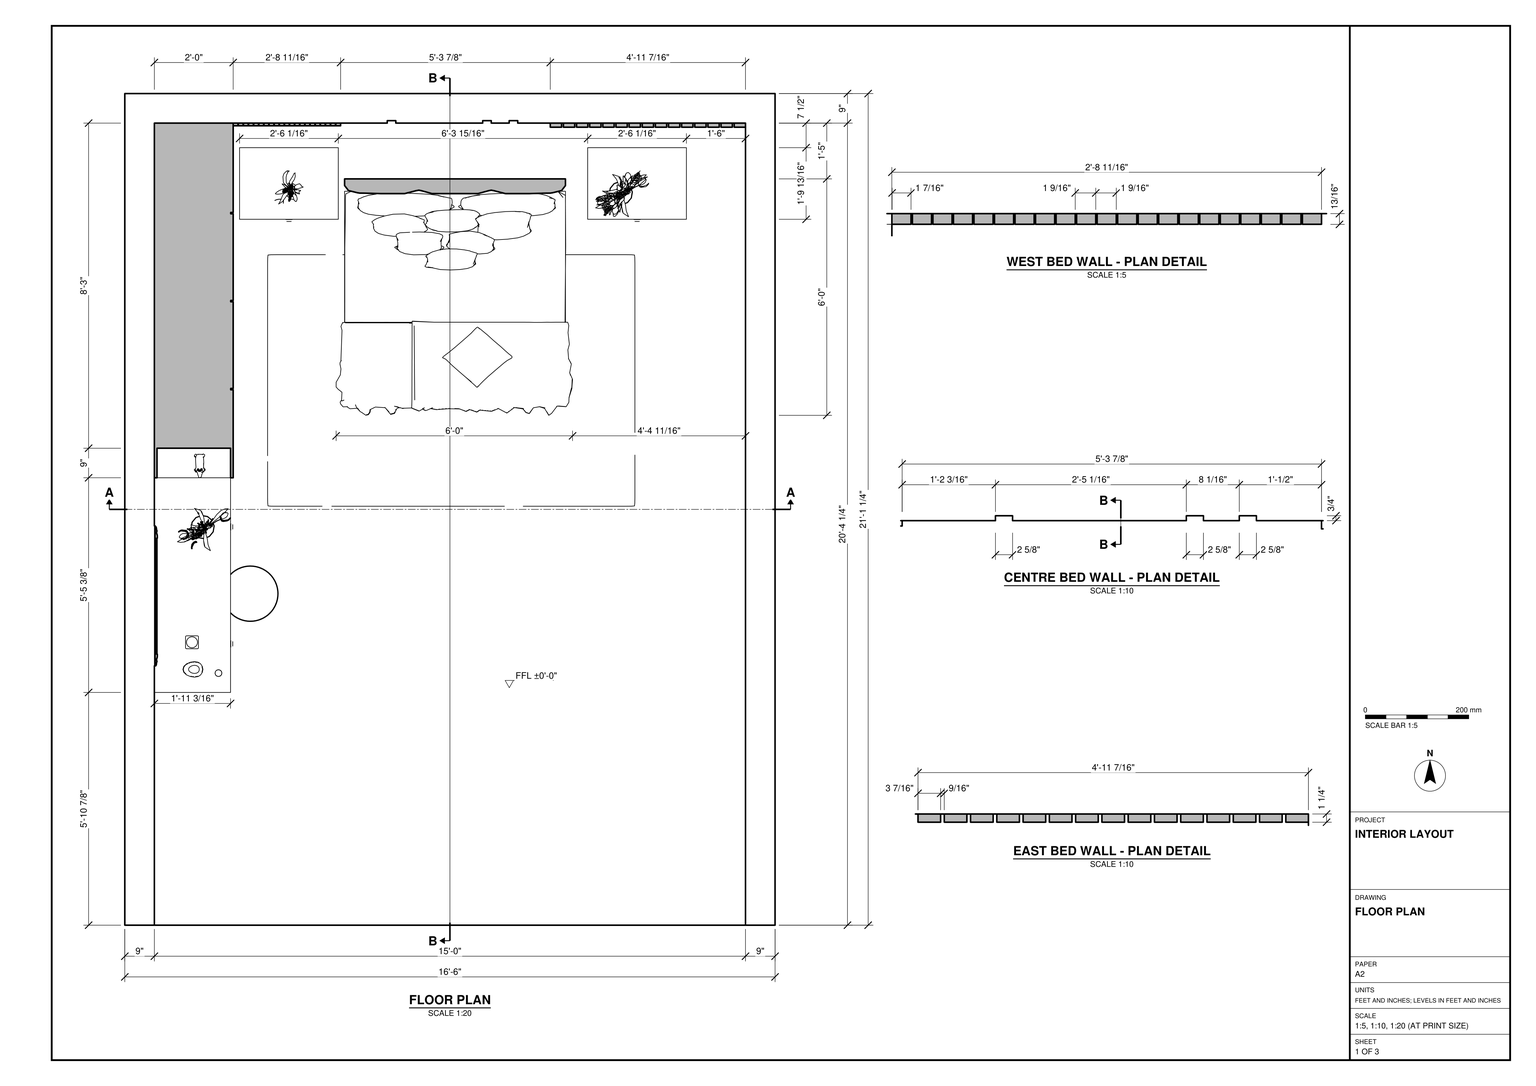
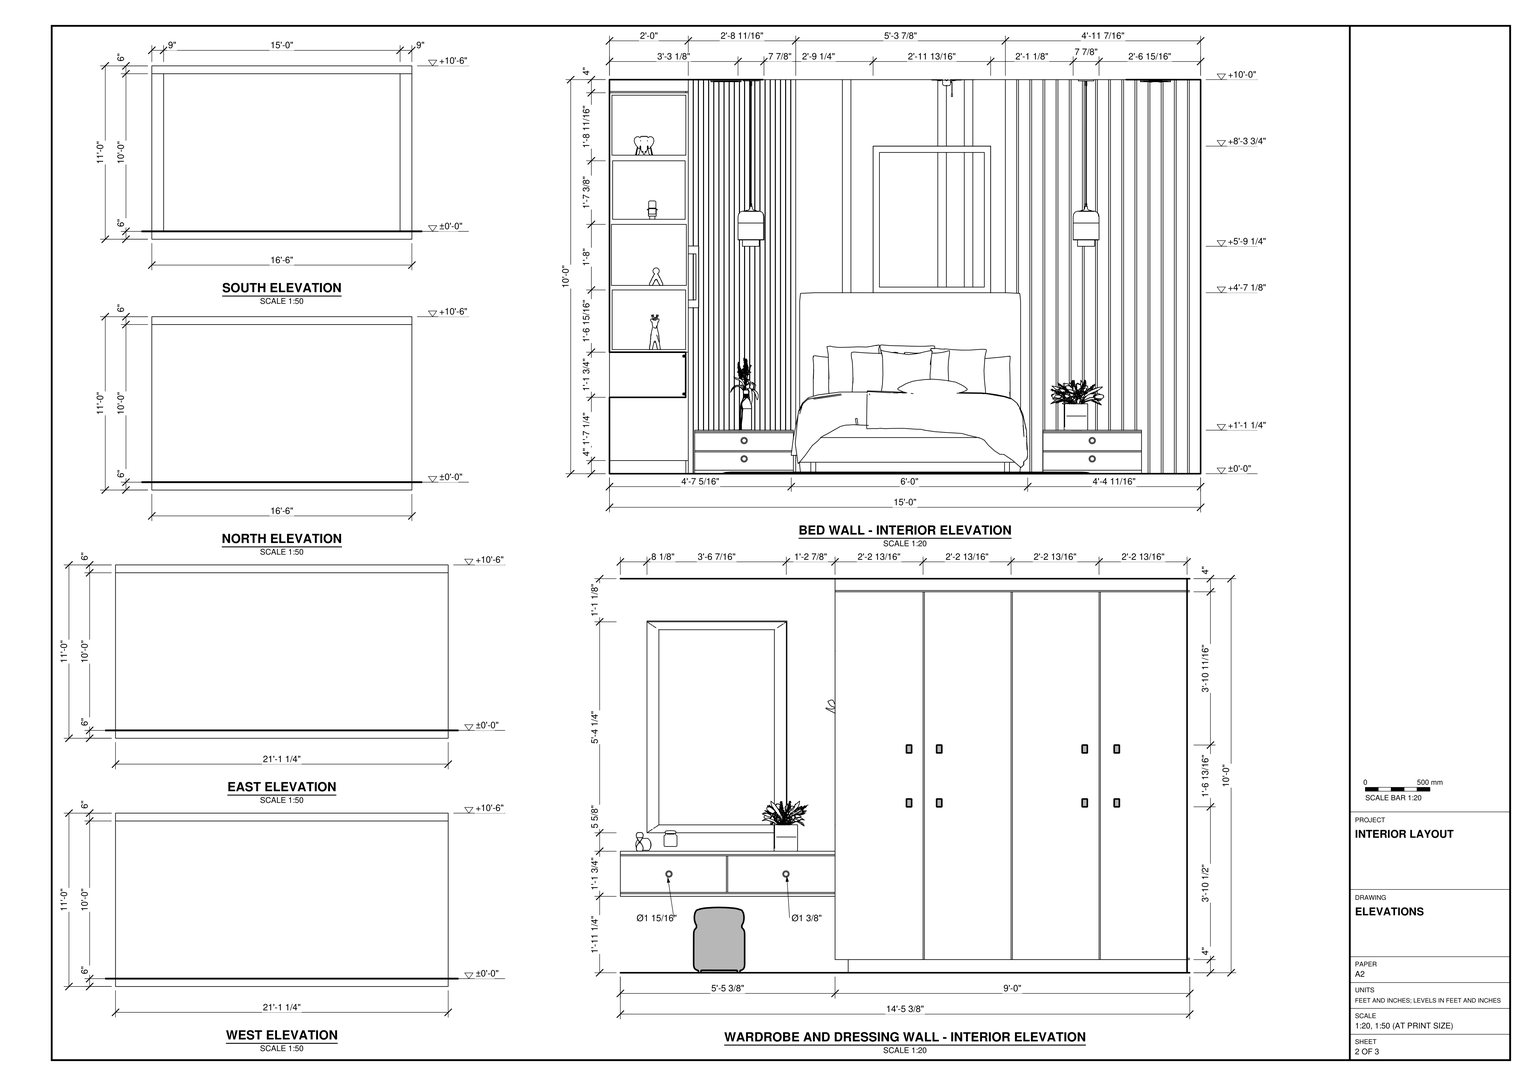
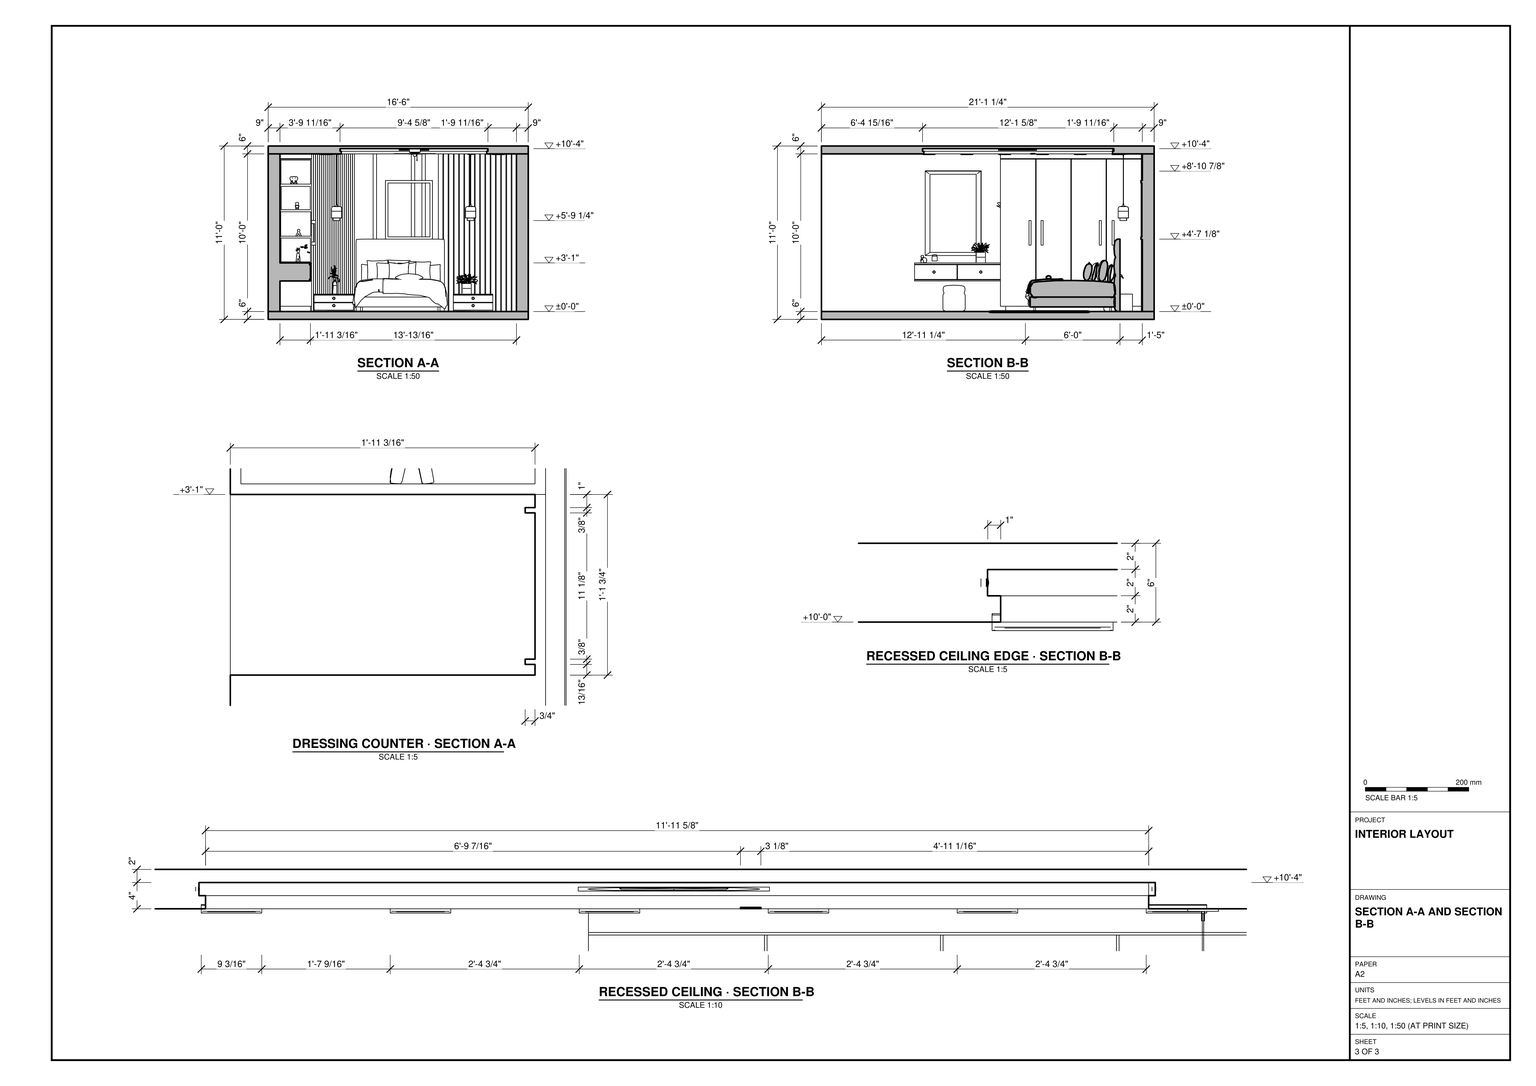
Model the bedroom in SketchUp from task_files/diagram_01.pdf. Work in feet and inches. The room shell measures 16'-6" across, 21'-1 1/4" from south to north and 11'-0" in overall height. Set the single finished floor at ±0'-0". Model the 9" walls on the north, east and west sides, leaving the south side open as shown in section. Include the 6" floor and roof slabs and form the stepped edge of the ceiling recess to match the section detail.

Place the bed with its headboard toward the north wall and a low drawer unit on either side. Use the bed-wall plan details to distinguish the closely spaced vertical strips on the west from the wider strips on the east. Model the central panel and its framed rectangular feature above the headboard. Along the west wall, build the tall wardrobe with its door fronts, handles and end display shelves. Continue the run toward the south with a wall-mounted dressing counter, drawers, a mirror above and a stool below. Keep the floor beyond the dressing area clear as shown in plan. Decor and loose items, including the rug, plants, pendant lights and shelf objects, may be any suitable library components.

Organise the walls, slabs and roof, and each furniture or joinery piece, as separate groups or components. Use components for repeated parts. Save one SketchUp model as output_files/bedroom_with_a_panelled_bed_wall_and_dressing_area.skp.

# SketchUp Ruby script. Lengths in inches.
U = 1.inch
M = Sketchup.active_model
def pt(a) = Geom::Point3d.new(a.map { |v| v * U })
def face(e, loops, mat)
  f = e.add_face(loops[0].map { |a| pt(a) })
  loops[1..].each { |l| e.add_face(l.map { |a| pt(a) }).erase! }
  f.material = f.back_material = mat if mat
  f
end
# faces: each face lists its corners as indices into pts; further lists are holes
def faces(e, pts, list, mat = nil) = list.each { |f| face(e, (f[0].is_a?(Array) ? f : [f]).map { |l| l.map { |i| pts[i] } }, mat) }
# xy, xz, yz: faces in a plane at the given z, y or x. An outline is a flat list of corners, or four numbers for a rectangle; further outlines are holes
def ring(l) = l.size == 4 ? [[l[0], l[1]], [l[2], l[1]], [l[2], l[3]], [l[0], l[3]]] : l.each_slice(2).to_a
def flat(e, list, mat, &to3) = list.each { |f| face(e, (f[0].is_a?(Array) ? f : [f]).map { |l| ring(l).map { |u, v| to3.(u, v) } }, mat) }
def xy(e, z, list, mat = nil) = flat(e, list, mat) { |x, y| [x, y, z] }
def xz(e, y, list, mat = nil) = flat(e, list, mat) { |x, z| [x, y, z] }
def yz(e, x, list, mat = nil) = flat(e, list, mat) { |y, z| [x, y, z] }
def lines(e, pts, list) = list.each { |a, b| e.add_line(pt(pts[a]), pt(pts[b])) }
# prism: a flat outline (further loops are holes) pulled along v
def prism(e, loops, v, mat = nil)
  f = face(e, loops, mat); d = Geom::Vector3d.new(v.map { |x| x * U })
  f.pushpull(f.normal.samedirection?(d) ? d.length : -d.length)
end
def box(e, o, s, mat = nil) = prism(e, [[o, [o[0] + s[0], o[1], o[2]], [o[0] + s[0], o[1] + s[1], o[2]], [o[0], o[1] + s[1], o[2]]]], [0, 0, s[2]], mat)
def at(x, y, z, deg = 0) = Geom::Transformation.translation(pt([x, y, z])) * Geom::Transformation.rotation(ORIGIN, Z_AXIS, deg.degrees)
def axes(o, x, y, z) = Geom::Transformation.new([*x, 0, *y, 0, *z, 0, *pt(o).to_a, 1])
def part(name) = M.definitions.add(name)
# library, detail: a bought-in or finely detailed component or shape, given as its bounding box
def library(name, o, s) = part(name).tap { |d| box(d.entities, o, s) }
def detail(e, o, s) = box(e.add_group.entities, o, s)
def put(e, d, t, mat = nil) = e.add_instance(d, t).tap { |i| i.material = mat if mat }
def group(e, t, mat = nil) = e.add_group.tap { |g| g.transformation = t; g.material = mat if mat }.entities
root = M.entities
M.materials.add("0210 AP 9427 DELICATE PINK").color = [242, 226, 232]
M.materials.add("0305 AP 7196 SOFT BALLAD").color = [223, 219, 224]
M.materials.add("0664 AP 2361 MEHENDI-N").color = [90, 109, 82]
M.materials.add("Emissive").color = [236, 231, 178]
M.materials.add("Emissive\#1").color = [231, 232, 187]
M.materials.add("Generic").color = [228, 229, 211]
M.materials.add("Gold 10k").color = [251, 232, 180]
M.materials.add("PDM_Stainless_Steel").color = [184, 186, 183]
M.materials.add("Tiles Simple 02 100cm").color = [183, 183, 183]
M.materials.add("[Color M07]").color = [58, 58, 58]
M.materials.add("[Wood Board Cork]").color = [215, 201, 115]
M.materials.add("[Wood Cherry Original]").color = [147, 83, 40]
c1 = library("Bed 003",[-38.05,-87.1,0],[75.86,87.1,55.12])
c2 = library("Pendant 114-21",[-3.95,-3.95,-50.75],[7.9,7.9,50.75])
c3 = part("Handle_13.skp\#1")
xy(c3.entities,-0.19,[[-2.31,-0.77,-2.31,0,-1.75,0,-1.75,-0.59,1.75,-0.59,1.75,0,2.31,0,2.31,-0.77]],"PDM_Stainless_Steel")
xy(c3.entities,0.19,[[-2.31,-0.77,2.31,-0.77,2.31,0,1.75,0,1.75,-0.59,-1.75,-0.59,-1.75,0,-2.31,0]],"PDM_Stainless_Steel")
xz(c3.entities,-0.79,[[-2.31,-0.18,2.31,0.18]],"PDM_Stainless_Steel")
xz(c3.entities,-0.57,[[-1.74,-0.18,1.74,0.18]],"PDM_Stainless_Steel")
yz(c3.entities,-2.33,[[-0.77,-0.18,0,0.18]],"PDM_Stainless_Steel")
yz(c3.entities,-1.74,[[-0.57,-0.18,0,0.18]],"PDM_Stainless_Steel")
yz(c3.entities,1.74,[[-0.57,-0.18,0,0.18]],"PDM_Stainless_Steel")
yz(c3.entities,2.33,[[-0.77,-0.18,0,0.18]],"PDM_Stainless_Steel")
p = [[-2.33,-0.77,-0.18],[-2.31,-0.79,-0.18],[-2.31,-0.79,0.18],[-2.33,-0.77,0.18],[-2.31,-0.77,-0.19],[-2.33,0,-0.18],
  [-2.31,0,-0.19],[2.31,-0.77,-0.19],[2.31,-0.79,-0.18],[2.33,-0.77,-0.18],[2.33,-0.77,0.18],[2.31,-0.79,0.18],
  [2.31,0,-0.19],[2.33,0,-0.18],[-1.74,0,-0.18],[-1.74,-0.57,-0.18],[-1.75,-0.59,-0.19],[-1.75,0,-0.19],
  [1.74,-0.57,-0.18],[1.75,-0.59,-0.19],[1.74,0,-0.18],[1.75,0,-0.19],[-2.31,-0.77,0.19],[-2.31,0,0.19],
  [-2.33,0,0.18],[2.31,-0.77,0.19],[2.33,0,0.18],[2.31,0,0.19],[-1.74,-0.57,0.18],[-1.74,0,0.18],
  [-1.75,0,0.19],[-1.75,-0.59,0.19],[1.74,-0.57,0.18],[1.75,-0.59,0.19],[1.74,0,0.18],[1.75,0,0.19]]
faces(c3.entities,p,[[0,1,2,3],[4,1,0],[5,6,4,0],[7,8,1,4],[8,9,10,11],[7,9,8],[12,13,9,7],[14,15,16,17],
  [15,18,19,16],[18,20,21,19],[3,22,23,24],[3,2,22],[11,25,22,2],[10,25,11],[26,27,25,10],[28,29,30,31],
  [32,28,31,33],[34,32,33,35]],"PDM_Stainless_Steel")
c4 = library("Tlon Light 650 Ceiling 152 007",[-12.8,-12.8,-3.78],[25.6,25.6,3.58])
c5 = library("Fan 90-20",[-15.86,-15.86,-9.19],[31.73,31.72,9.19])
c6 = library("Group\#3",[-131.71,-139.42,-0.73],[161.77,161.23,107.59])
c7 = library("Group\#4",[-0.5,-0.5,0],[112.59,1,2])
c8 = library("Group\#5",[-0.5,-0.5,0],[1,145.59,2])
c9 = library("Group\#6",[-0.5,-0.5,0],[113.59,1,2])
c10 = library("Group\#7",[-0.5,-0.5,0],[1,146.59,2])
xy(root,-6,[[0,0,198,253.25]])
xy(root,0,[[0,0,9,0,9,244.25,79.91,244.25,79.91,245,82.52,245,82.52,244.25,108.97,244.25,108.97,245,111.58,245,111.58,244.25,117.04,244.25,117.04,245,119.64,245,119.64,244.25,189,244.25,189,0,198,0,198,253.25,0,253.25],[9,140.25,32.25,244.25]])
xy(root,0,[[9,0,189,0,189,244.25,119.64,244.25,119.64,245,117.04,245,117.04,244.25,111.58,244.25,111.58,245,108.97,245,108.97,244.25,82.52,244.25,82.52,245,79.91,245,79.91,244.25,32.25,244.25,32.25,140.25,9,140.25]],"Tiles Simple 02 100cm")
xy(root,4,[[9,136.25,33,140.25],[32.25,140.25,33,163.05],[32.25,163.45,33,189.84],[32.25,190.24,33,216.64],[32.25,217.04,33,243.4375],
  [32.25,243.4375,33,244.25]])
xy(root,23.25,[[9,70.875,32.2,136.25]],"Generic")
xy(root,24.0625,[[31.45,70.875,32.2,136.25]],"[Color M07]")
xy(root,24.46,[[31.45,70.875,32.2,103.16],[31.45,103.5625,32.2,136.25]],"[Color M07]")
xy(root,35.6,[[31.45,70.875,32.2,103.16],[31.45,103.5625,32.2,136.25]],"[Color M07]")
xy(root,36,[[31.45,70.875,32.2,136.25]],"[Color M07]")
xy(root,37,[[9,70.875,32.2,136.25]],"Generic")
xy(root,37.8,[[9.8,136.25,32.2,145.25]],"Generic")
xy(root,42.62,[[9,78.98,9.24,121.6]],"Emissive\#1")
xy(root,54.88,[[89.27,243.25,108.97,244.25],[108.97,243.25,111.58,244.25],[111.58,243.25,117.04,244.25],[117.04,243.25,119.64,244.25],[119.64,243.25,125.08,244.25]],"[Wood Board Cork]")
xy(root,55.95,[[9.8,144.25,32.2,145.25]],"Emissive")
xy(root,55.95,[[9.8,136.25,32.2,144.25]],"Generic")
xy(root,56.82,[[91.2,243.25,108.97,243.9375],[108.97,243.25,111.58,243.9375],[111.58,243.25,117.04,243.9375],[117.04,243.25,119.64,243.9375],[119.64,243.25,123.15,243.9375]])
xy(root,57.34,[[9.59,136.25,32.41,145.25]],"Generic")
xy(root,75.91,[[9.59,144.25,32.41,145.25]],"Emissive")
xy(root,75.91,[[9.59,136.25,32.41,144.25]],"Generic")
xy(root,77.46,[[9.96,136.25,32.04,145.25]],"Generic")
xy(root,95.29,[[9.96,144.25,32.04,145.25]],"Emissive")
xy(root,95.29,[[9.96,136.25,32.04,144.25]],"Generic")
xy(root,96.99,[[9.74,136.25,32.26,145.25]],"Generic")
xy(root,97.82,[[91.2,243.25,108.97,243.9375],[108.97,243.25,111.58,243.9375],[111.58,243.25,117.04,243.9375],[117.04,243.25,119.64,243.9375],[119.64,243.25,123.15,243.9375]],"[Wood Board Cork]")
xy(root,99.76,[[89.27,243.25,108.97,244.25],[108.97,243.25,111.58,244.25],[111.58,243.25,117.04,244.25],[117.04,243.25,119.64,244.25],[119.64,243.25,125.08,244.25]],"[Wood Board Cork]")
xy(root,107.12,[[9,78.98,9.24,121.6]],"Emissive\#1")
xy(root,115.26,[[9.74,144.25,32.26,145.25]],"Emissive")
xy(root,115.26,[[9.74,136.25,32.26,144.25]],"Generic")
xy(root,116,[[32.25,243.4375,33,244.25]])
xy(root,116,[[32.25,136.25,33,163.05],[32.25,163.45,33,189.84],[32.25,190.24,33,216.64],[32.25,217.04,33,243.4375]],"[Color M07]")
xy(root,116.4,[[32.25,136.25,33,244.25]],"[Color M07]")
xy(root,120,[[0,0,0,253.25,198,253.25,198,0,189,0,189,244.25,119.64,244.25,119.64,245,117.04,245,117.04,244.25,111.58,244.25,111.58,245,108.97,245,108.97,244.25,82.52,244.25,82.52,245,79.91,245,79.91,244.25,9,244.25,9,0],[9,136.25,33,244.25]])
xy(root,120,[[[9,0,9,136.25,33,136.25,33,244.25,79.91,244.25,79.91,245,82.52,245,82.52,244.25,108.97,244.25,108.97,245,111.58,245,111.58,244.25,117.04,244.25,117.04,245,119.64,245,119.64,244.25,189,244.25,189,0],[55.7,77.95,166.3,221.55]]],"0305 AP 7196 SOFT BALLAD")
xy(root,122,[[54.7,76.95,167.3,77.95],[54.7,77.95,55.7,222.55],[166.3,77.95,167.3,221.55],[55.7,221.55,167.3,222.55]])
xy(root,124,[[54.7,76.95,167.3,222.55]],"0305 AP 7196 SOFT BALLAD")
xy(root,126,[[0,0,198,253.25]])
xz(root,0,[[0,-6,198,0],[0,0,9,120],[9,0,189,120],[189,0,198,120],[0,120,198,126]])
xz(root,70.875,[[9,23.25,32.2,23.25,32.2,24.0625,31.45,24.0625,31.45,24.46,32.2,24.46,32.2,35.6,31.45,35.6,31.45,36,32.2,36,32.2,37,9,37]],"Generic")
xz(root,76.95,[[166.3,122,167.3,124]])
xz(root,77.95,[[55.7,120,166.3,122]])
xz(root,78.98,[[9,42.62,9.24,107.12]],"Emissive\#1")
xz(root,103.16,[[31.45,24.46,32.2,35.6]],"[Color M07]")
xz(root,103.5625,[[31.45,24.46,32.2,35.6]],"[Color M07]")
xz(root,121.6,[[9,42.62,9.24,107.12]],"Emissive\#1")
xz(root,136.25,[[9,23.25,32.2,23.25,32.2,24.0625,31.45,24.0625,31.45,24.46,32.2,24.46,32.2,35.6,31.45,35.6,31.45,36,32.2,36,32.2,37,9,37]])
xz(root,136.25,[[9,4,33,4,33,37,32.2,37,32.2,36,31.45,36,31.45,35.6,32.2,35.6,32.2,24.46,31.45,24.46,31.45,24.0625,32.2,24.0625,32.2,23.25,9,23.25],[[9,37,33,116],[9.59,57.34,32.41,75.91],[9.74,96.99,32.26,115.26],[9.8,37.8,32.2,55.95],[9.96,77.46,32.04,95.29]],[9,116.4,33,120]],"Generic")
xz(root,136.25,[[9,116,32.25,116.4]],"[Color M07]")
xz(root,140.25,[[9,0,32.25,4]],"Generic")
xz(root,145.25,[[9.8,37.8,32.2,55.95],[9.59,57.34,32.41,75.91],[9.96,77.46,32.04,95.29],[9.74,96.99,32.26,115.26]],"Generic")
xz(root,163.05,[[32.25,4,33,37]])
xz(root,163.05,[[32.25,37,33,116]],"[Color M07]")
xz(root,163.45,[[32.25,4,33,37]])
xz(root,163.45,[[32.25,37,33,116]],"[Color M07]")
xz(root,189.84,[[32.25,4,33,37]])
xz(root,189.84,[[32.25,37,33,116]],"[Color M07]")
xz(root,190.24,[[32.25,4,33,37]])
xz(root,190.24,[[32.25,37,33,116]],"[Color M07]")
xz(root,216.64,[[32.25,4,33,37]])
xz(root,216.64,[[32.25,37,33,116]],"[Color M07]")
xz(root,217.04,[[32.25,4,33,37]])
xz(root,217.04,[[32.25,37,33,116]],"[Color M07]")
xz(root,221.55,[[55.7,120,166.3,122]],"0305 AP 7196 SOFT BALLAD")
xz(root,243.25,[[[89.27,54.88,125.08,99.76],[89.29,54.9,125.0625,99.74]]])
xz(root,243.25,[[[89.29,54.9,125.0625,99.74],[91.2,56.82,123.15,97.82]]],"[Wood Board Cork]")
xz(root,243.9375,[[91.2,56.82,123.15,97.82]],"[Wood Cherry Original]")
xz(root,244.25,[[9,0,32.25,0,32.25,4,33,4,33,116,32.25,116,32.25,116.4,33,116.4,33,120,9,120],[111.58,0,117.04,54.88],[108.97,54.88,111.58,99.76],[117.04,54.88,119.64,99.76]])
xz(root,244.25,[[34.46,0,79.91,120],[82.52,0,108.97,0,108.97,54.88,89.27,54.88,89.27,99.76,108.97,99.76,108.97,120,82.52,120],[119.64,0,185.56,0,185.56,120,119.64,120,119.64,99.76,125.08,99.76,125.08,54.88,119.64,54.88],[111.58,99.76,117.04,120]],"0305 AP 7196 SOFT BALLAD")
xz(root,245,[[79.91,0,82.52,120],[108.97,0,111.58,120],[117.04,0,119.64,120]],"Gold 10k")
xz(root,253.25,[[0,-6,198,0],[0,0,198,120],[0,120,198,126]])
yz(root,0,[[0,-6,253.25,0],[0,0,253.25,120],[0,120,253.25,126]])
yz(root,9,[[140.25,0,244.25,0,244.25,120,136.25,120,136.25,4,140.25,4]])
yz(root,9,[[[0,0,140.25,0,140.25,4,136.25,4,136.25,23.25,70.875,23.25,70.875,37,136.25,37,136.25,120,0,120],[78.98,42.62,121.6,107.12]]],"0664 AP 2361 MEHENDI-N")
yz(root,9.24,[[78.98,42.62,121.6,107.12]])
yz(root,9.59,[[136.25,57.34,145.25,75.91]],"Generic")
yz(root,9.74,[[136.25,96.99,145.25,115.26]],"Generic")
yz(root,9.8,[[136.25,37.8,145.25,55.95]],"Generic")
yz(root,9.96,[[136.25,77.46,145.25,95.29]],"Generic")
yz(root,31.45,[[70.875,24.0625,136.25,24.46],[103.16,24.46,103.5625,35.6],[70.875,35.6,136.25,36]],"[Color M07]")
yz(root,32.04,[[136.25,77.46,145.25,95.29]],"Generic")
yz(root,32.2,[[70.875,23.25,136.25,24.0625],[70.875,24.46,103.16,35.6],[103.5625,24.46,136.25,35.6],[70.875,36,136.25,37],[136.25,37.8,145.25,55.95]],"Generic")
yz(root,32.25,[[140.25,0,244.25,4]],"Generic")
yz(root,32.25,[[163.05,4,163.45,116],[189.84,4,190.24,116],[216.64,4,217.04,116],[136.25,116,244.25,116.4]],"[Color M07]")
yz(root,32.26,[[136.25,96.99,145.25,115.26]],"Generic")
yz(root,32.41,[[136.25,57.34,145.25,75.91]],"Generic")
yz(root,33,[[243.4375,4,244.25,116]])
yz(root,33,[[136.25,4,163.05,116],[163.45,4,189.84,116],[190.24,4,216.64,116],[217.04,4,243.4375,116],[136.25,116.4,244.25,120]],"Generic")
yz(root,54.7,[[221.55,122,222.55,124]])
yz(root,55.7,[[77.95,120,221.55,122]],"0305 AP 7196 SOFT BALLAD")
yz(root,79.91,[[244.25,0,245,120]],"Gold 10k")
yz(root,82.52,[[244.25,0,245,120]],"Gold 10k")
yz(root,89.27,[[243.25,54.88,244.25,99.76]],"[Wood Board Cork]")
yz(root,91.2,[[243.25,56.82,243.9375,97.82]],"[Wood Board Cork]")
yz(root,108.97,[[244.25,0,245,120]],"Gold 10k")
yz(root,111.58,[[244.25,0,245,120]],"Gold 10k")
yz(root,117.04,[[244.25,0,245,120]],"Gold 10k")
yz(root,119.64,[[244.25,0,245,120]],"Gold 10k")
yz(root,123.15,[[243.25,56.82,243.9375,97.82]],"[Wood Board Cork]")
yz(root,125.08,[[243.25,54.88,244.25,99.76]],"[Wood Board Cork]")
yz(root,166.3,[[77.95,120,221.55,122]],"0305 AP 7196 SOFT BALLAD")
yz(root,189,[[0,0,244.25,120]],"0305 AP 7196 SOFT BALLAD")
yz(root,198,[[0,-6,253.25,0],[0,0,253.25,120],[0,120,253.25,126]])
put(root,c1,axes([100.46,227.26,0],[0.94908,0,0],[0,0.82665,0],[0,0,1]))
put(root,c2,at(52.09,229.83,120))
put(root,c3,axes([33,158.78,59.93],[0,0,-4.04319],[-4.04319,0,0],[0,4.04319,0]))
put(root,c3,axes([33,167.97,59.93],[0,0,-4.04319],[-4.04319,0,0],[0,4.04319,0]))
put(root,c3,axes([33,212.28,59.93],[0,0,-4.04319],[-4.04319,0,0],[0,4.04319,0]))
put(root,c3,axes([33,222.03,59.93],[0,0,-4.04319],[-4.04319,0,0],[0,4.04319,0]))
put(root,c2,at(154.13,229.83,120))
put(root,c4,axes([44.46,81.9,120.71],[0.36,0,0],[0,0.36,0],[0,0,0.36]))
put(root,c4,axes([44.46,110.68,120.71],[0.36,0,0],[0,0.36,0],[0,0,0.36]))
put(root,c4,axes([44.46,139.45,120.71],[0.36,0,0],[0,0.36,0],[0,0,0.36]))
put(root,c4,axes([44.46,168.23,120.71],[0.36,0,0],[0,0.36,0],[0,0,0.36]))
put(root,c4,axes([44.46,197,120.71],[0.36,0,0],[0,0.36,0],[0,0,0.36]))
put(root,c4,axes([44.46,225.78,120.71],[0.36,0,0],[0,0.36,0],[0,0,0.36]))
put(root,c4,axes([175.27,81.9,120.71],[0.36,0,0],[0,0.36,0],[0,0,0.36]))
put(root,c4,axes([175.27,109.5,120.71],[0.36,0,0],[0,0.36,0],[0,0,0.36]))
put(root,c4,axes([175.27,137.1,120.71],[0.36,0,0],[0,0.36,0],[0,0,0.36]))
put(root,c4,axes([175.27,164.7,120.71],[0.36,0,0],[0,0.36,0],[0,0,0.36]))
put(root,c4,axes([175.27,192.3,120.71],[0.36,0,0],[0,0.36,0],[0,0,0.36]))
put(root,c4,axes([175.27,219.9,120.71],[0.36,0,0],[0,0.36,0],[0,0,0.36]))
put(root,c4,axes([115.54,230.66,121.32],[0.36,0,0],[0,0.36,0],[0,0,0.36]))
put(root,c5,at(111.63,160.95,124))
g1 = group(root,at(185.56,244.25,0))
xy(g1,0,[[-56,-1.25,-52.56,0],[-52,-1.25,-48.56,0],[-48,-1.25,-44.56,0],[-44,-1.25,-40.56,0],[-40,-1.25,-36.56,0],
  [-36,-1.25,-32.56,0],[-32,-1.25,-28.56,0],[-28,-1.25,-24.56,0],[-24,-1.25,-20.56,0],[-20,-1.25,-16.56,0],
  [-16,-1.25,-12.56,0],[-12,-1.25,-8.56,0],[-8,-1.25,-4.56,0],[-4,-1.25,-0.56,0],[0,-1.25,3.44,0]])
xy(g1,120,[[-56,-1.25,-52.56,0],[-52,-1.25,-48.56,0],[-48,-1.25,-44.56,0],[-44,-1.25,-40.56,0],[-40,-1.25,-36.56,0],
  [-36,-1.25,-32.56,0],[-32,-1.25,-28.56,0],[-28,-1.25,-24.56,0],[-24,-1.25,-20.56,0],[-20,-1.25,-16.56,0],
  [-16,-1.25,-12.56,0],[-12,-1.25,-8.56,0],[-8,-1.25,-4.56,0],[-4,-1.25,-0.56,0],[0,-1.25,3.44,0]])
xz(g1,-1.25,[[-56,0,-52.56,120],[-52,0,-48.56,120],[-48,0,-44.56,120],[-44,0,-40.56,120],[-40,0,-36.56,120],
  [-36,0,-32.56,120],[-32,0,-28.56,120],[-28,0,-24.56,120],[-24,0,-20.56,120],[-20,0,-16.56,120],
  [-16,0,-12.56,120],[-12,0,-8.56,120],[-8,0,-4.56,120],[-4,0,-0.56,120],[0,0,3.44,120]],"0210 AP 9427 DELICATE PINK")
xz(g1,0,[[-56,0,-52.56,120],[-52,0,-48.56,120],[-48,0,-44.56,120],[-44,0,-40.56,120],[-40,0,-36.56,120],
  [-36,0,-32.56,120],[-32,0,-28.56,120],[-28,0,-24.56,120],[-24,0,-20.56,120],[-20,0,-16.56,120],
  [-16,0,-12.56,120],[-12,0,-8.56,120],[-8,0,-4.56,120],[-4,0,-0.56,120],[0,0,3.44,120]])
yz(g1,-56,[[-1.25,0,0,120]],"0210 AP 9427 DELICATE PINK")
yz(g1,-52.56,[[-1.25,0,0,120]])
yz(g1,-52,[[-1.25,0,0,120]],"0210 AP 9427 DELICATE PINK")
yz(g1,-48.56,[[-1.25,0,0,120]])
yz(g1,-48,[[-1.25,0,0,120]],"0210 AP 9427 DELICATE PINK")
yz(g1,-44.56,[[-1.25,0,0,120]])
yz(g1,-44,[[-1.25,0,0,120]],"0210 AP 9427 DELICATE PINK")
yz(g1,-40.56,[[-1.25,0,0,120]])
yz(g1,-40,[[-1.25,0,0,120]],"0210 AP 9427 DELICATE PINK")
yz(g1,-36.56,[[-1.25,0,0,120]])
yz(g1,-36,[[-1.25,0,0,120]],"0210 AP 9427 DELICATE PINK")
yz(g1,-32.56,[[-1.25,0,0,120]])
yz(g1,-32,[[-1.25,0,0,120]],"0210 AP 9427 DELICATE PINK")
yz(g1,-28.56,[[-1.25,0,0,120]])
yz(g1,-28,[[-1.25,0,0,120]],"0210 AP 9427 DELICATE PINK")
yz(g1,-24.56,[[-1.25,0,0,120]])
yz(g1,-24,[[-1.25,0,0,120]],"0210 AP 9427 DELICATE PINK")
yz(g1,-20.56,[[-1.25,0,0,120]])
yz(g1,-20,[[-1.25,0,0,120]],"0210 AP 9427 DELICATE PINK")
yz(g1,-16.56,[[-1.25,0,0,120]])
yz(g1,-16,[[-1.25,0,0,120]],"0210 AP 9427 DELICATE PINK")
yz(g1,-12.56,[[-1.25,0,0,120]])
yz(g1,-12,[[-1.25,0,0,120]],"0210 AP 9427 DELICATE PINK")
yz(g1,-8.56,[[-1.25,0,0,120]])
yz(g1,-8,[[-1.25,0,0,120]],"0210 AP 9427 DELICATE PINK")
yz(g1,-4.56,[[-1.25,0,0,120]])
yz(g1,-4,[[-1.25,0,0,120]],"0210 AP 9427 DELICATE PINK")
yz(g1,-0.56,[[-1.25,0,0,120]])
yz(g1,0,[[-1.25,0,0,120]],"0210 AP 9427 DELICATE PINK")
yz(g1,3.44,[[-1.25,0,0,120]])
g2 = group(root,at(33,244.25,0))
xy(g2,0,[[0,-0.8125,1.46,0],[1.5625,-0.8125,3.02,0],[3.125,-0.8125,4.58,0],[4.6875,-0.8125,6.15,0],[6.25,-0.8125,7.71,0],
  [7.8125,-0.8125,9.27,0],[9.375,-0.8125,10.83,0],[10.9375,-0.8125,12.4,0],[12.5,-0.8125,13.96,0],[14.0625,-0.8125,15.52,0],
  [15.625,-0.8125,17.08,0],[17.1875,-0.8125,18.65,0],[18.75,-0.8125,20.21,0],[20.3125,-0.8125,21.77,0],[21.875,-0.8125,23.33,0],
  [23.4375,-0.8125,24.9,0],[25,-0.8125,26.46,0],[26.5625,-0.8125,28.02,0],[28.125,-0.8125,29.58,0],[29.6875,-0.8125,31.15,0],
  [31.25,-0.8125,32.71,0]])
xy(g2,120,[[0,-0.8125,1.46,0],[1.5625,-0.8125,3.02,0],[3.125,-0.8125,4.58,0],[4.6875,-0.8125,6.15,0],[6.25,-0.8125,7.71,0],
  [7.8125,-0.8125,9.27,0],[9.375,-0.8125,10.83,0],[10.9375,-0.8125,12.4,0],[12.5,-0.8125,13.96,0],[14.0625,-0.8125,15.52,0],
  [15.625,-0.8125,17.08,0],[17.1875,-0.8125,18.65,0],[18.75,-0.8125,20.21,0],[20.3125,-0.8125,21.77,0],[21.875,-0.8125,23.33,0],
  [23.4375,-0.8125,24.9,0],[25,-0.8125,26.46,0],[26.5625,-0.8125,28.02,0],[28.125,-0.8125,29.58,0],[29.6875,-0.8125,31.15,0],
  [31.25,-0.8125,32.71,0]])
xz(g2,-0.8125,[[0,0,1.46,120],[1.5625,0,3.02,120],[3.125,0,4.58,120],[4.6875,0,6.15,120],[6.25,0,7.71,120],
  [7.8125,0,9.27,120],[9.375,0,10.83,120],[10.9375,0,12.4,120],[12.5,0,13.96,120],[14.0625,0,15.52,120],
  [15.625,0,17.08,120],[17.1875,0,18.65,120],[18.75,0,20.21,120],[20.3125,0,21.77,120],[21.875,0,23.33,120],
  [23.4375,0,24.9,120],[25,0,26.46,120],[26.5625,0,28.02,120],[28.125,0,29.58,120],[29.6875,0,31.15,120],
  [31.25,0,32.71,120]],"[Wood Cherry Original]")
xz(g2,0,[[0,0,1.46,120],[1.5625,0,3.02,120],[3.125,0,4.58,120],[4.6875,0,6.15,120],[6.25,0,7.71,120],
  [7.8125,0,9.27,120],[9.375,0,10.83,120],[10.9375,0,12.4,120],[12.5,0,13.96,120],[14.0625,0,15.52,120],
  [15.625,0,17.08,120],[17.1875,0,18.65,120],[18.75,0,20.21,120],[20.3125,0,21.77,120],[21.875,0,23.33,120],
  [23.4375,0,24.9,120],[25,0,26.46,120],[26.5625,0,28.02,120],[28.125,0,29.58,120],[29.6875,0,31.15,120],
  [31.25,0,32.71,120]])
yz(g2,0,[[-0.8125,0,0,4],[-0.8125,4,0,4.4],[-0.8125,4.4,0,116],[-0.8125,116,0,116.4],[-0.8125,116.4,0,120]])
yz(g2,1.46,[[-0.8125,0,0,120]],"[Wood Cherry Original]")
yz(g2,1.5625,[[-0.8125,0,0,4],[-0.8125,4,0,4.4],[-0.8125,4.4,0,116],[-0.8125,116,0,116.4],[-0.8125,116.4,0,120]])
yz(g2,3.02,[[-0.8125,0,0,120]],"[Wood Cherry Original]")
yz(g2,3.125,[[-0.8125,0,0,4],[-0.8125,4,0,4.4],[-0.8125,4.4,0,116],[-0.8125,116,0,116.4],[-0.8125,116.4,0,120]])
yz(g2,4.58,[[-0.8125,0,0,120]],"[Wood Cherry Original]")
yz(g2,4.6875,[[-0.8125,0,0,4],[-0.8125,4,0,4.4],[-0.8125,4.4,0,116],[-0.8125,116,0,116.4],[-0.8125,116.4,0,120]])
yz(g2,6.15,[[-0.8125,0,0,120]],"[Wood Cherry Original]")
yz(g2,6.25,[[-0.8125,0,0,4],[-0.8125,4,0,4.4],[-0.8125,4.4,0,116],[-0.8125,116,0,116.4],[-0.8125,116.4,0,120]])
yz(g2,7.71,[[-0.8125,0,0,120]],"[Wood Cherry Original]")
yz(g2,7.8125,[[-0.8125,0,0,4],[-0.8125,4,0,4.4],[-0.8125,4.4,0,116],[-0.8125,116,0,116.4],[-0.8125,116.4,0,120]])
yz(g2,9.27,[[-0.8125,0,0,120]],"[Wood Cherry Original]")
yz(g2,9.375,[[-0.8125,0,0,4],[-0.8125,4,0,4.4],[-0.8125,4.4,0,116],[-0.8125,116,0,116.4],[-0.8125,116.4,0,120]])
yz(g2,10.83,[[-0.8125,0,0,120]],"[Wood Cherry Original]")
yz(g2,10.9375,[[-0.8125,0,0,4],[-0.8125,4,0,4.4],[-0.8125,4.4,0,116],[-0.8125,116,0,116.4],[-0.8125,116.4,0,120]])
yz(g2,12.4,[[-0.8125,0,0,120]],"[Wood Cherry Original]")
yz(g2,12.5,[[-0.8125,0,0,4],[-0.8125,4,0,4.4],[-0.8125,4.4,0,116],[-0.8125,116,0,116.4],[-0.8125,116.4,0,120]])
yz(g2,13.96,[[-0.8125,0,0,120]],"[Wood Cherry Original]")
yz(g2,14.0625,[[-0.8125,0,0,4],[-0.8125,4,0,4.4],[-0.8125,4.4,0,116],[-0.8125,116,0,116.4],[-0.8125,116.4,0,120]])
yz(g2,15.52,[[-0.8125,0,0,120]],"[Wood Cherry Original]")
yz(g2,15.625,[[-0.8125,0,0,4],[-0.8125,4,0,4.4],[-0.8125,4.4,0,116],[-0.8125,116,0,116.4],[-0.8125,116.4,0,120]])
yz(g2,17.08,[[-0.8125,0,0,120]],"[Wood Cherry Original]")
yz(g2,17.1875,[[-0.8125,0,0,4],[-0.8125,4,0,4.4],[-0.8125,4.4,0,116],[-0.8125,116,0,116.4],[-0.8125,116.4,0,120]])
yz(g2,18.65,[[-0.8125,0,0,120]],"[Wood Cherry Original]")
yz(g2,18.75,[[-0.8125,0,0,4],[-0.8125,4,0,4.4],[-0.8125,4.4,0,116],[-0.8125,116,0,116.4],[-0.8125,116.4,0,120]])
yz(g2,20.21,[[-0.8125,0,0,120]],"[Wood Cherry Original]")
yz(g2,20.3125,[[-0.8125,0,0,4],[-0.8125,4,0,4.4],[-0.8125,4.4,0,116],[-0.8125,116,0,116.4],[-0.8125,116.4,0,120]])
yz(g2,21.77,[[-0.8125,0,0,120]],"[Wood Cherry Original]")
yz(g2,21.875,[[-0.8125,0,0,4],[-0.8125,4,0,4.4],[-0.8125,4.4,0,116],[-0.8125,116,0,116.4],[-0.8125,116.4,0,120]])
yz(g2,23.33,[[-0.8125,0,0,120]],"[Wood Cherry Original]")
yz(g2,23.4375,[[-0.8125,0,0,4],[-0.8125,4,0,4.4],[-0.8125,4.4,0,116],[-0.8125,116,0,116.4],[-0.8125,116.4,0,120]])
yz(g2,24.9,[[-0.8125,0,0,120]],"[Wood Cherry Original]")
yz(g2,25,[[-0.8125,0,0,4],[-0.8125,4,0,4.4],[-0.8125,4.4,0,116],[-0.8125,116,0,116.4],[-0.8125,116.4,0,120]])
yz(g2,26.46,[[-0.8125,0,0,120]],"[Wood Cherry Original]")
yz(g2,26.5625,[[-0.8125,0,0,4],[-0.8125,4,0,4.4],[-0.8125,4.4,0,116],[-0.8125,116,0,116.4],[-0.8125,116.4,0,120]])
yz(g2,28.02,[[-0.8125,0,0,120]],"[Wood Cherry Original]")
yz(g2,28.125,[[-0.8125,0,0,4],[-0.8125,4,0,4.4],[-0.8125,4.4,0,116],[-0.8125,116,0,116.4],[-0.8125,116.4,0,120]])
yz(g2,29.58,[[-0.8125,0,0,120]],"[Wood Cherry Original]")
yz(g2,29.6875,[[-0.8125,0,0,4],[-0.8125,4,0,4.4],[-0.8125,4.4,0,116],[-0.8125,116,0,116.4],[-0.8125,116.4,0,120]])
yz(g2,31.15,[[-0.8125,0,0,120]],"[Wood Cherry Original]")
yz(g2,31.25,[[-0.8125,0,0,4],[-0.8125,4,0,4.4],[-0.8125,4.4,0,116],[-0.8125,116,0,116.4],[-0.8125,116.4,0,120]])
yz(g2,32.71,[[-0.8125,0,0,120]],"[Wood Cherry Original]")
put(root,c6,at(140.94,214.96,0))
put(root,c7,at(54.7,76.95,122))
put(root,c8,at(54.7,76.95,122))
put(root,c9,at(54.7,222.55,122))
put(root,c10,at(167.3,76.95,122))
